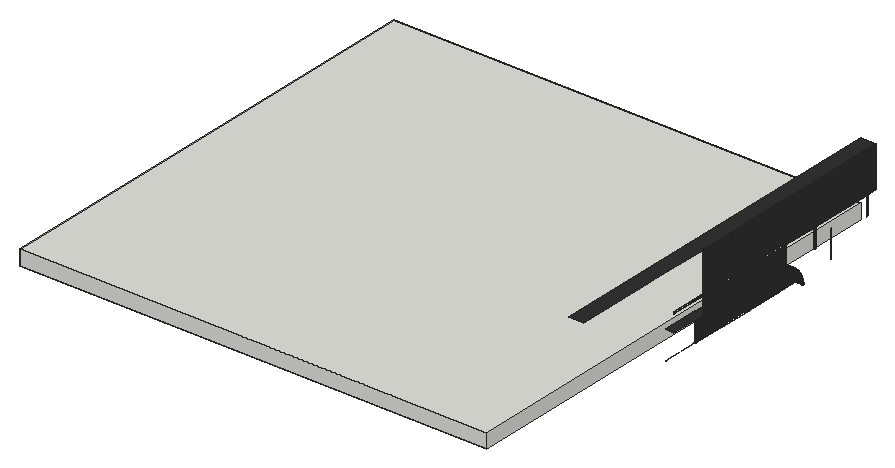
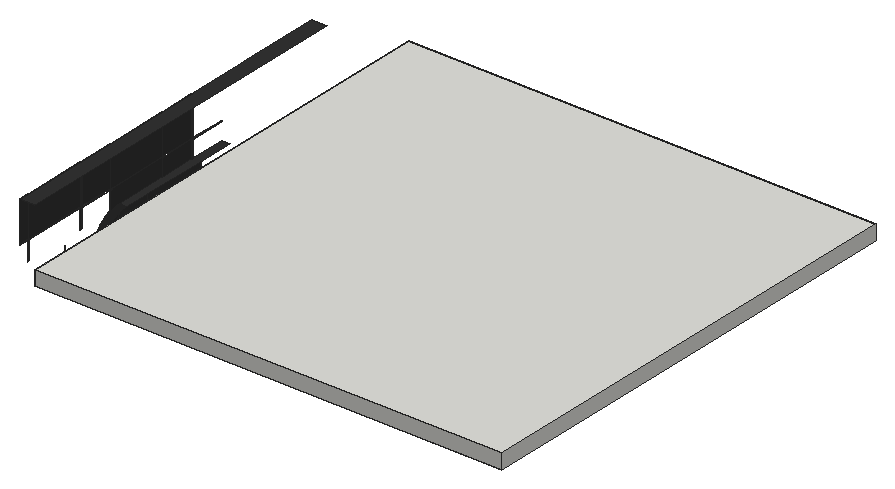
# SketchUp Ruby script. Lengths in inches.
U = 1.inch
M = Sketchup.active_model
def pt(a) = Geom::Point3d.new(a.map { |v| v * U })
def face(e, loops, mat)
  f = e.add_face(loops[0].map { |a| pt(a) })
  loops[1..].each { |l| e.add_face(l.map { |a| pt(a) }).erase! }
  f.material = f.back_material = mat if mat
  f
end
# faces: each face lists its corners as indices into pts; further lists are holes
def faces(e, pts, list, mat = nil) = list.each { |f| face(e, (f[0].is_a?(Array) ? f : [f]).map { |l| l.map { |i| pts[i] } }, mat) }
# xy, xz, yz: faces in a plane at the given z, y or x. An outline is a flat list of corners, or four numbers for a rectangle; further outlines are holes
def ring(l) = l.size == 4 ? [[l[0], l[1]], [l[2], l[1]], [l[2], l[3]], [l[0], l[3]]] : l.each_slice(2).to_a
def flat(e, list, mat, &to3) = list.each { |f| face(e, (f[0].is_a?(Array) ? f : [f]).map { |l| ring(l).map { |u, v| to3.(u, v) } }, mat) }
def xy(e, z, list, mat = nil) = flat(e, list, mat) { |x, y| [x, y, z] }
def xz(e, y, list, mat = nil) = flat(e, list, mat) { |x, z| [x, y, z] }
def yz(e, x, list, mat = nil) = flat(e, list, mat) { |y, z| [x, y, z] }
def lines(e, pts, list) = list.each { |a, b| e.add_line(pt(pts[a]), pt(pts[b])) }
# prism: a flat outline (further loops are holes) pulled along v
def prism(e, loops, v, mat = nil)
  f = face(e, loops, mat); d = Geom::Vector3d.new(v.map { |x| x * U })
  f.pushpull(f.normal.samedirection?(d) ? d.length : -d.length)
end
def box(e, o, s, mat = nil) = prism(e, [[o, [o[0] + s[0], o[1], o[2]], [o[0] + s[0], o[1] + s[1], o[2]], [o[0], o[1] + s[1], o[2]]]], [0, 0, s[2]], mat)
def at(x, y, z, deg = 0) = Geom::Transformation.translation(pt([x, y, z])) * Geom::Transformation.rotation(ORIGIN, Z_AXIS, deg.degrees)
def axes(o, x, y, z) = Geom::Transformation.new([*x, 0, *y, 0, *z, 0, *pt(o).to_a, 1])
def part(name) = M.definitions.add(name)
# library, detail: a bought-in or finely detailed component or shape, given as its bounding box
def library(name, o, s) = part(name).tap { |d| box(d.entities, o, s) }
def detail(e, o, s) = box(e.add_group.entities, o, s)
def put(e, d, t, mat = nil) = e.add_instance(d, t).tap { |i| i.material = mat if mat }
def group(e, t, mat = nil) = e.add_group.tap { |g| g.transformation = t; g.material = mat if mat }.entities
root = M.entities
M.materials.add("[Granite Dark Gray]").color = [51, 50, 50]
xy(root,378,[[436.875,424,437,477],[436.875,478,437,507],[436.875,508,437,526.17]],"[Granite Dark Gray]")
xy(root,379,[[436.875,393,437,423],[436.875,424,437,477],[436.875,478,437,507],[436.875,508,437,525.99]],"[Granite Dark Gray]")
xy(root,402,[[437,393,437,423,436.875,423,436.875,424,437,424,437,477,436.875,477,436.875,478,437,478,437,498,444,498,444,454,443.875,454,443.875,453,444,453,444,424,443.875,424,443.875,423,444,423,444,393],[437,498,444,498.27],[437,498.27,444,498.53]],"[Granite Dark Gray]")
xy(root,416,[[443.875,393,444,423],[443.875,424,444,453],[443.875,454,444,507],[443.875,508,444,537],[443.875,538,444,591],
  [443.875,592,444,600]],"[Granite Dark Gray]")
xy(root,417,[[443.875,393,444,423],[443.875,424,444,453],[443.875,454,444,507],[443.875,508,444,537],[443.875,538,444,591],
  [443.875,592,444,600]],"[Granite Dark Gray]")
xy(root,450,[[432,300,444,300,444,369,443.875,369,443.875,370,444,370,444,423,443.875,423,443.875,424,444,424,444,453,443.875,453,443.875,454,444,454,444,507,443.875,507,443.875,508,444,508,444,537,443.875,537,443.875,538,444,538,444,591,443.875,591,443.875,592,444,592,444,600,432,600]],"[Granite Dark Gray]")
xz(root,423,[[436.875,379,437,402],[443.875,402,444,416],[443.875,417,444,450]],"[Granite Dark Gray]")
xz(root,424,[[436.875,379,437,402],[443.875,402,444,416],[443.875,417,444,450]],"[Granite Dark Gray]")
xz(root,453,[[443.875,402,444,416],[443.875,417,444,450]],"[Granite Dark Gray]")
xz(root,454,[[443.875,402,444,416],[443.875,417,444,450]],"[Granite Dark Gray]")
xz(root,477,[[436.875,379,437,402]],"[Granite Dark Gray]")
xz(root,478,[[436.875,379,437,402]],"[Granite Dark Gray]")
xz(root,507,[[436.875,379,437,400.54],[443.875,400.54,444,402],[443.875,402,444,416],[443.875,417,444,450]],"[Granite Dark Gray]")
xz(root,508,[[436.875,379,437,400.19],[443.875,400.19,444,402],[443.875,402,444,416],[443.875,417,444,450]],"[Granite Dark Gray]")
xz(root,537,[[443.875,400.54,444,402],[443.875,402,444,416],[443.875,417,444,450]],"[Granite Dark Gray]")
xz(root,538,[[443.875,400.19,444,402],[443.875,402,444,416],[443.875,417,444,450]],"[Granite Dark Gray]")
xz(root,591,[[443.875,400.54,444,402],[443.875,402,444,416],[443.875,417,444,450]],"[Granite Dark Gray]")
xz(root,592,[[443.875,400.19,444,402],[443.875,402,444,416],[443.875,417,444,450]],"[Granite Dark Gray]")
yz(root,437,[[424,379,477,402],[478,379,507,379,507,400.54,506.9,400.58,506.64,400.66,506.39,400.74,506.13,400.82,505.88,400.89,505.62,400.96,505.37,401.03,504.85,401.17,504.07,401.35,503.8125,401.4,503.55,401.45,503.29,401.51,503.03,401.55,502.77,401.6,502.5,401.64,501.98,401.72,501.71,401.76,501.45,401.79,501.1875,401.82,500.92,401.85,500.66,401.875,500.39,401.9,500.125,401.92,499.86,401.9375,499.6,401.96,499.33,401.97,499.0625,401.98,498.8,401.99,498.53,402,478,402],[508,379,525.99,379,525.96,379.14,525.91,379.4,525.73,380.18,525.67,380.4375,525.6,380.69,525.46,381.21,525.39,381.46,525.31,381.72,525.24,381.97,525.16,382.23,525.07,382.48,524.99,382.73,524.9,382.98,524.8125,383.23,524.72,383.48,524.53,383.98,524.43,384.23,524.33,384.47,524.22,384.72,524.12,384.96,524.01,385.2,523.9,385.45,523.78,385.6875,523.67,385.93,523.55,386.17,523.43,386.4,523.3125,386.64,523.0625,387.11,522.93,387.34,522.67,387.8,522.53,388.03,522.4,388.26,522.26,388.49,522.12,388.71,521.97,388.9375,521.83,389.16,521.23,390.04,521.07,390.26,520.43,391.1,520.26,391.3125,520.1,391.52,519.93,391.72,519.76,391.93,519.58,392.13,519.41,392.33,519.05,392.73,518.87,392.92,518.69,393.12,518.51,393.31,518.32,393.5,517.94,393.875,517.75,394.06,517.56,394.24,517.36,394.42,517.17,394.6,516.77,394.96,516.37,395.3,516.16,395.47,515.96,395.64,515.75,395.81,515.54,395.97,515.33,396.14,515.12,396.3,514.9,396.45,514.6875,396.61,514.47,396.77,514.03,397.07,513.8125,397.22,513.59,397.36,513.37,397.51,513.14,397.65,512.92,397.79,512.69,397.93,512.46,398.0625,512.23,398.2,511.77,398.46,511.53,398.59,511.3,398.71,511.0625,398.83,510.83,398.95,510.35,399.19,510.11,399.3,509.87,399.42,509.625,399.52,509.38,399.63,509.14,399.74,508.64,399.94,508.4,400.04,508.15,400.13,508,400.19]],"[Granite Dark Gray]")
yz(root,444,[[507,400.54,507,416,454,416,454,402,498.53,402,498.8,401.99,499.0625,401.98,499.33,401.97,499.6,401.96,499.86,401.9375,500.125,401.92,500.39,401.9,500.66,401.875,500.92,401.85,501.1875,401.82,501.45,401.79,501.71,401.76,501.98,401.72,502.5,401.64,502.77,401.6,503.03,401.55,503.29,401.51,503.55,401.45,503.8125,401.4,504.07,401.35,504.85,401.17,505.37,401.03,505.62,400.96,505.88,400.89,506.13,400.82,506.39,400.74,506.64,400.66,506.9,400.58],[424,402,453,416],[424,417,453,450],[454,417,507,450],[508,417,537,450],
  [538,417,591,450],[592,417,600,450]],"[Granite Dark Gray]")
p = [[444,526.11,378.35],[444,526.07,378.62],[436.875,526.07,378.62],[436.875,526.11,378.35],[444,526.02,378.88],[436.875,526.02,378.88],
  [444,525.96,379.14],[437,525.96,379.14],[437,525.99,379],[436.875,525.99,379],[444,525.91,379.4],[437,525.91,379.4],
  [444,525.85,379.66],[437,525.85,379.66],[444,525.79,379.92],[437,525.79,379.92],[444,525.73,380.18],[437,525.73,380.18],
  [444,525.67,380.4375],[437,525.67,380.4375],[444,525.6,380.69],[437,525.6,380.69],[444,525.53,380.95],[437,525.53,380.95],
  [444,525.46,381.21],[437,525.46,381.21],[444,525.39,381.46],[437,525.39,381.46],[444,525.31,381.72],[437,525.31,381.72],
  [444,525.24,381.97],[437,525.24,381.97],[444,525.16,382.23],[437,525.16,382.23],[444,525.07,382.48],[437,525.07,382.48],
  [444,524.99,382.73],[437,524.99,382.73],[444,524.9,382.98],[437,524.9,382.98],[444,524.8125,383.23],[437,524.8125,383.23],
  [444,524.72,383.48],[437,524.72,383.48],[444,524.625,383.73],[437,524.625,383.73],[444,524.53,383.98],[437,524.53,383.98],
  [444,524.43,384.23],[437,524.43,384.23],[444,524.33,384.47],[437,524.33,384.47],[444,524.22,384.72],[437,524.22,384.72],
  [444,524.12,384.96],[437,524.12,384.96],[444,524.01,385.2],[437,524.01,385.2],[444,523.9,385.45],[437,523.9,385.45],
  [444,523.78,385.6875],[437,523.78,385.6875],[444,523.67,385.93],[437,523.67,385.93],[444,523.55,386.17],[437,523.55,386.17],
  [444,523.43,386.4],[437,523.43,386.4],[444,523.3125,386.64],[437,523.3125,386.64],[444,523.1875,386.875],[437,523.1875,386.875],
  [444,523.0625,387.11],[437,523.0625,387.11],[444,522.93,387.34],[437,522.93,387.34],[444,522.8,387.57],[437,522.8,387.57],
  [444,522.67,387.8],[437,522.67,387.8],[444,522.53,388.03],[437,522.53,388.03],[444,522.4,388.26],[437,522.4,388.26],
  [444,522.26,388.49],[437,522.26,388.49],[444,522.12,388.71],[437,522.12,388.71],[444,521.97,388.9375],[437,521.97,388.9375],
  [444,521.83,389.16],[437,521.83,389.16],[444,521.68,389.38],[437,521.68,389.38],[444,521.53,389.6],[437,521.53,389.6],
  [444,521.38,389.82],[437,521.38,389.82],[444,521.23,390.04],[437,521.23,390.04],[444,521.07,390.26],[437,521.07,390.26],
  [444,520.91,390.47],[437,520.91,390.47],[444,520.75,390.68],[437,520.75,390.68],[444,520.59,390.89],[437,520.59,390.89],
  [444,520.43,391.1],[437,520.43,391.1],[444,520.26,391.3125],[437,520.26,391.3125],[444,520.1,391.52],[437,520.1,391.52],
  [444,519.93,391.72],[437,519.93,391.72],[444,519.76,391.93],[437,519.76,391.93],[444,519.58,392.13],[437,519.58,392.13],
  [444,519.41,392.33],[437,519.41,392.33],[444,519.23,392.53],[437,519.23,392.53],[444,519.05,392.73],[437,519.05,392.73],
  [444,518.87,392.92],[437,518.87,392.92],[444,518.69,393.12],[437,518.69,393.12],[444,518.51,393.31],[437,518.51,393.31],
  [444,518.32,393.5],[437,518.32,393.5],[444,518.13,393.6875],[437,518.13,393.6875],[444,517.94,393.875],[437,517.94,393.875],
  [444,517.75,394.06],[437,517.75,394.06],[444,517.56,394.24],[437,517.56,394.24],[444,517.36,394.42],[437,517.36,394.42],
  [444,517.17,394.6],[437,517.17,394.6],[444,516.97,394.78],[437,516.97,394.78],[444,516.77,394.96],[437,516.77,394.96],
  [444,516.57,395.13],[437,516.57,395.13],[444,516.37,395.3],[437,516.37,395.3],[444,516.16,395.47],[437,516.16,395.47],
  [444,515.96,395.64],[437,515.96,395.64],[444,515.75,395.81],[437,515.75,395.81],[444,515.54,395.97],[437,515.54,395.97],
  [444,515.33,396.14],[437,515.33,396.14],[444,515.12,396.3],[437,515.12,396.3],[444,514.9,396.45],[437,514.9,396.45],
  [444,514.6875,396.61],[437,514.6875,396.61],[444,514.47,396.77],[437,514.47,396.77],[444,514.25,396.92],[437,514.25,396.92],
  [444,514.03,397.07],[437,514.03,397.07],[444,513.8125,397.22],[437,513.8125,397.22],[444,513.59,397.36],[437,513.59,397.36],
  [444,513.37,397.51],[437,513.37,397.51],[444,513.14,397.65],[437,513.14,397.65],[444,512.92,397.79],[437,512.92,397.79],
  [444,512.69,397.93],[437,512.69,397.93],[444,512.46,398.0625],[437,512.46,398.0625],[444,512.23,398.2],[437,512.23,398.2],
  [444,512,398.33],[437,512,398.33],[444,511.77,398.46],[437,511.77,398.46],[444,511.53,398.59],[437,511.53,398.59],
  [444,511.3,398.71],[437,511.3,398.71],[444,511.0625,398.83],[437,511.0625,398.83],[444,510.83,398.95],[437,510.83,398.95],
  [444,510.59,399.07],[437,510.59,399.07],[444,510.35,399.19],[437,510.35,399.19],[444,510.11,399.3],[437,510.11,399.3],
  [444,509.87,399.42],[437,509.87,399.42],[444,509.625,399.52],[437,509.625,399.52],[444,509.38,399.63],[437,509.38,399.63],
  [444,509.14,399.74],[437,509.14,399.74],[444,508.89,399.84],[437,508.89,399.84],[444,508.64,399.94],[437,508.64,399.94],
  [444,508.4,400.04],[437,508.4,400.04],[444,508.15,400.13],[437,508.15,400.13],[444,508,400.19],[443.875,508,400.19],
  [443.875,507.9,400.23],[436.875,507.9,400.23],[436.875,508,400.19],[437,508,400.19],[443.875,507.65,400.32],[436.875,507.65,400.32],
  [443.875,507.4,400.41],[436.875,507.4,400.41],[443.875,507.15,400.49],[436.875,507.15,400.49],[444,507,400.54],[444,506.9,400.58],
  [437,506.9,400.58],[437,507,400.54],[436.875,507,400.54],[443.875,507,400.54],[444,506.64,400.66],[437,506.64,400.66],
  [444,506.39,400.74],[444,506.13,400.82],[437,506.13,400.82],[437,506.39,400.74],[444,505.88,400.89],[437,505.88,400.89],
  [444,505.62,400.96],[437,505.62,400.96],[444,505.37,401.03],[444,505.11,401.1],[437,505.11,401.1],[437,505.37,401.03],
  [444,504.85,401.17],[437,504.85,401.17],[444,504.59,401.23],[444,504.33,401.29],[437,504.33,401.29],[437,504.59,401.23],
  [444,504.07,401.35],[444,503.8125,401.4],[437,503.8125,401.4],[437,504.07,401.35],[444,503.55,401.45],[437,503.55,401.45],
  [444,503.29,401.51],[444,503.03,401.55],[437,503.03,401.55],[437,503.29,401.51],[444,502.5,401.64],[444,502.24,401.68],
  [437,502.24,401.68],[437,502.5,401.64],[444,502.77,401.6],[437,502.77,401.6],[444,501.98,401.72],[444,501.71,401.76],
  [437,501.71,401.76],[437,501.98,401.72],[444,501.1875,401.82],[444,500.92,401.85],[437,500.92,401.85],[437,501.1875,401.82],
  [444,501.45,401.79],[437,501.45,401.79],[444,499.86,401.9375],[444,499.6,401.96],[437,499.6,401.96],[437,499.86,401.9375],
  [444,500.125,401.92],[437,500.125,401.92],[444,500.39,401.9],[437,500.39,401.9],[444,500.66,401.875],[437,500.66,401.875],
  [444,498.8,401.99],[444,498.53,402],[437,498.53,402],[437,498.8,401.99],[444,499.0625,401.98],[437,499.0625,401.98],
  [444,499.33,401.97],[437,499.33,401.97],[437,526.17,379],[437,507,402],[437,508,402],[437,508,400.54],
  [437,562,400.54],[437,562,400.19],[437,562,402],[437,562,379],[437,563,400.54],[437,563,400.19],
  [437,563,402],[437,563,379]]
faces(root,p,[[0,1,2,3],[1,4,5,2],[4,6,7,8,9,5],[6,10,11,7],[10,12,13,11],[12,14,15,13],[14,16,17,15],[16,18,19,17],
  [18,20,21,19],[20,22,23,21],[22,24,25,23],[24,26,27,25],[26,28,29,27],[28,30,31,29],[30,32,33,31],[32,34,35,33],
  [34,36,37,35],[36,38,39,37],[38,40,41,39],[40,42,43,41],[42,44,45,43],[44,46,47,45],[46,48,49,47],[48,50,51,49],
  [50,52,53,51],[52,54,55,53],[54,56,57,55],[56,58,59,57],[58,60,61,59],[60,62,63,61],[62,64,65,63],[64,66,67,65],
  [66,68,69,67],[68,70,71,69],[70,72,73,71],[72,74,75,73],[74,76,77,75],[76,78,79,77],[78,80,81,79],[80,82,83,81],
  [82,84,85,83],[84,86,87,85],[86,88,89,87],[88,90,91,89],[90,92,93,91],[92,94,95,93],[94,96,97,95],[96,98,99,97],
  [98,100,101,99],[100,102,103,101],[102,104,105,103],[104,106,107,105],[106,108,109,107],[108,110,111,109],[110,112,113,111],[112,114,115,113],
  [114,116,117,115],[116,118,119,117],[118,120,121,119],[120,122,123,121],[122,124,125,123],[124,126,127,125],[126,128,129,127],[128,130,131,129],
  [130,132,133,131],[132,134,135,133],[134,136,137,135],[136,138,139,137],[138,140,141,139],[140,142,143,141],[142,144,145,143],[144,146,147,145],
  [146,148,149,147],[148,150,151,149],[150,152,153,151],[152,154,155,153],[154,156,157,155],[156,158,159,157],[158,160,161,159],[160,162,163,161],
  [162,164,165,163],[164,166,167,165],[166,168,169,167],[168,170,171,169],[170,172,173,171],[172,174,175,173],[174,176,177,175],[176,178,179,177],
  [178,180,181,179],[180,182,183,181],[182,184,185,183],[184,186,187,185],[186,188,189,187],[188,190,191,189],[190,192,193,191],[192,194,195,193],
  [194,196,197,195],[196,198,199,197],[198,200,201,199],[200,202,203,201],[202,204,205,203],[204,206,207,205],[206,208,209,207],[208,210,211,209],
  [210,212,213,211],[212,214,215,213],[214,216,217,215],[216,218,219,217],[218,220,221,219],[220,222,223,221],[222,224,225,223],[224,226,227,228,229,230,231,225],
  [229,228,232,233],[233,232,234,235],[235,234,236,237],[238,239,240,241,242,237,236,243],[239,244,245,240],[246,247,248,249],[244,246,249,245],[247,250,251,248],
  [250,252,253,251],[254,255,256,257],[252,254,257,253],[255,258,259,256],[260,261,262,263],[258,260,263,259],[264,265,266,267],[261,264,267,262],
  [265,268,269,266],[270,271,272,273],[268,270,273,269],[274,275,276,277],[278,274,277,279],[271,278,279,272],[280,281,282,283],[275,280,283,276],
  [284,285,286,287],[288,284,287,289],[281,288,289,282],[290,291,292,293],[294,290,293,295],[296,294,295,297],[298,296,297,299],[285,298,299,286],
  [300,301,302,303],[304,300,303,305],[306,304,305,307],[291,306,307,292]],"[Granite Dark Gray]")
lines(root,p,[[308,8],[309,241],[310,311],[311,231],[312,313],[314,312],[313,315],[316,317],[318,316],[317,319]])
g1 = group(root,at(57,225,390))
box(g1,[-9,-9,0],[384,384,12])
